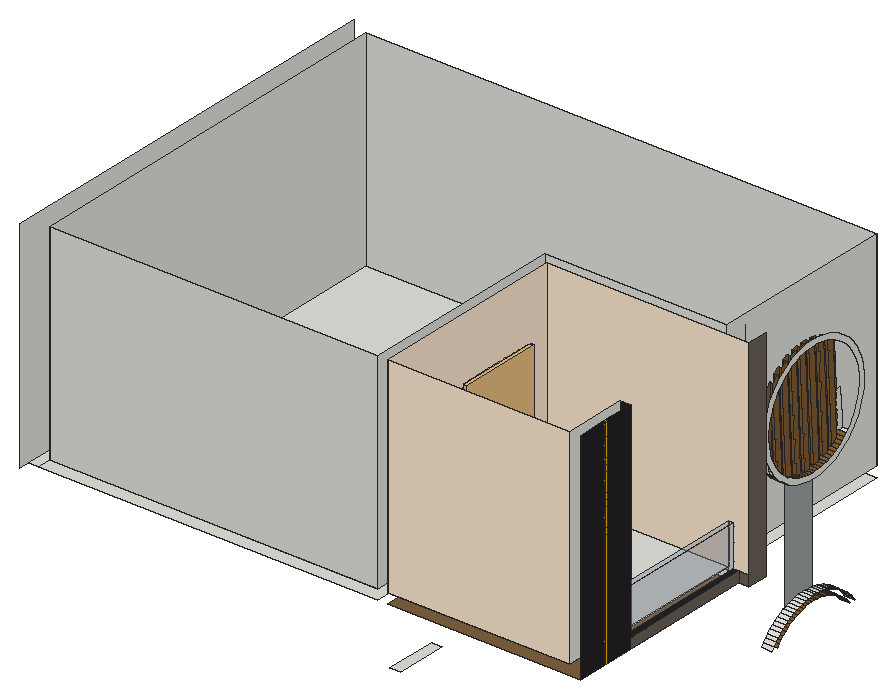
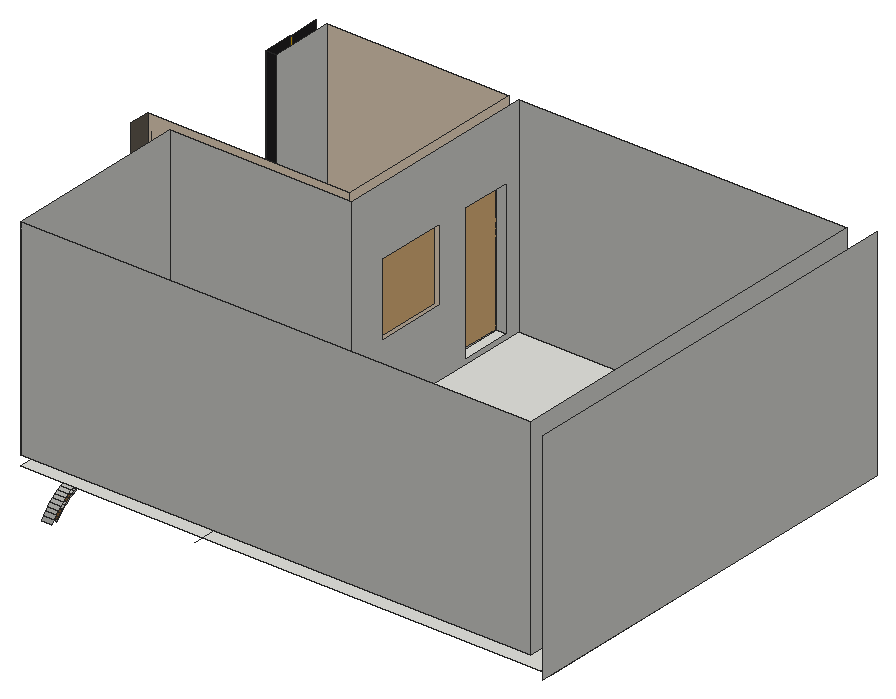
# SketchUp Ruby script. Lengths in inches.
U = 1.inch
M = Sketchup.active_model
def pt(a) = Geom::Point3d.new(a.map { |v| v * U })
def face(e, loops, mat)
  f = e.add_face(loops[0].map { |a| pt(a) })
  loops[1..].each { |l| e.add_face(l.map { |a| pt(a) }).erase! }
  f.material = f.back_material = mat if mat
  f
end
# faces: each face lists its corners as indices into pts; further lists are holes
def faces(e, pts, list, mat = nil) = list.each { |f| face(e, (f[0].is_a?(Array) ? f : [f]).map { |l| l.map { |i| pts[i] } }, mat) }
# xy, xz, yz: faces in a plane at the given z, y or x. An outline is a flat list of corners, or four numbers for a rectangle; further outlines are holes
def ring(l) = l.size == 4 ? [[l[0], l[1]], [l[2], l[1]], [l[2], l[3]], [l[0], l[3]]] : l.each_slice(2).to_a
def flat(e, list, mat, &to3) = list.each { |f| face(e, (f[0].is_a?(Array) ? f : [f]).map { |l| ring(l).map { |u, v| to3.(u, v) } }, mat) }
def xy(e, z, list, mat = nil) = flat(e, list, mat) { |x, y| [x, y, z] }
def xz(e, y, list, mat = nil) = flat(e, list, mat) { |x, z| [x, y, z] }
def yz(e, x, list, mat = nil) = flat(e, list, mat) { |y, z| [x, y, z] }
def lines(e, pts, list) = list.each { |a, b| e.add_line(pt(pts[a]), pt(pts[b])) }
# prism: a flat outline (further loops are holes) pulled along v
def prism(e, loops, v, mat = nil)
  f = face(e, loops, mat); d = Geom::Vector3d.new(v.map { |x| x * U })
  f.pushpull(f.normal.samedirection?(d) ? d.length : -d.length)
end
def box(e, o, s, mat = nil) = prism(e, [[o, [o[0] + s[0], o[1], o[2]], [o[0] + s[0], o[1] + s[1], o[2]], [o[0], o[1] + s[1], o[2]]]], [0, 0, s[2]], mat)
def at(x, y, z, deg = 0) = Geom::Transformation.translation(pt([x, y, z])) * Geom::Transformation.rotation(ORIGIN, Z_AXIS, deg.degrees)
def axes(o, x, y, z) = Geom::Transformation.new([*x, 0, *y, 0, *z, 0, *pt(o).to_a, 1])
def part(name) = M.definitions.add(name)
# library, detail: a bought-in or finely detailed component or shape, given as its bounding box
def library(name, o, s) = part(name).tap { |d| box(d.entities, o, s) }
def detail(e, o, s) = box(e.add_group.entities, o, s)
def put(e, d, t, mat = nil) = e.add_instance(d, t).tap { |i| i.material = mat if mat }
def group(e, t, mat = nil) = e.add_group.tap { |g| g.transformation = t; g.material = mat if mat }.entities
root = M.entities
M.materials.add("C03_Honey_Glow").color = [255, 234, 209]
M.materials.add("C08_Toffee_Ember").color = [130, 92, 50]
M.materials.add("D05_Goldenrod_Hue").color = [255, 191, 0]
M.materials.add("Denim_03_1K").color = [156, 160, 160]
M.materials.add("Glass_Basic_01").color = [161, 173, 186]
M.materials["Glass_Basic_01"].alpha = 0.25
M.materials.add("Marble_07_1K").color = [36, 34, 36]
M.materials.add("Plaster_04_1K").color = [106, 98, 87]
M.materials.add("Plywood_01_1K").color = [125, 96, 64]
c1 = library("porta+4",[0.2,-5.42,1.33],[46.55,4.72,83.21])
c2 = library("mesh-165",[-1596.32,-2661.67,-39.91],[1702.88,1739.15,82.5])
c3 = part("Group15")
put(c3.entities,c2,at(294.66,859.51,3.5))
xy(root,213,[[206.5,30,212.5,60],[206.5,78,212.5,120]])
xy(root,252,[[5.5,21,11.5,135],[11.5,21,206.5,249],[317.82,101.57,320.5,104.14],[317.82,106.71,320.5,109.29],[317.82,111.86,320.5,114.43],
  [317.5,117,320.5,119.57],[317.5,122.14,320.5,124.71],[317.5,127.29,320.5,129.86],[317.5,132.43,320.5,135],[5.5,135,11.5,249],
  [206.5,135,317.5,141],[206.5,141,311.5,249]])
xy(root,252,[[[212.5,21,212.5,135,317.5,135,317.5,132.43,320.5,132.43,320.5,135,323.5,135,323.5,21],[317.82,101.57,320.5,101.57,320.5,104.14,317.82,104.14,317.82,106.71,320.5,106.71,320.5,109.29,317.82,109.29,317.82,111.86,320.5,111.86,320.5,114.43,317.82,114.43],[317.5,127.29,320.5,129.86],[317.5,122.14,320.5,124.71],[317.5,117,320.5,119.57]]],"Plywood_01_1K")
xy(root,258,[[17.5,21,206.67,21,206.67,141,311.5,141,311.5,249,17.5,249],[212.67,21,317.5,135]])
xy(root,258,[[320.5,57,323.5,135]],"Marble_07_1K")
xy(root,261,[[206.67,30,212.67,60]])
xy(root,282,[[317.5,57,320.5,135]],"Glass_Basic_01")
xz(root,21,[[17.5,258,206.67,378]])
xz(root,21,[[212.67,258,317.5,378]],"C03_Honey_Glow")
xz(root,30,[[206.67,261,212.67,339]])
xz(root,57,[[320.5,258,323.5,282],[317.5,282,323.5,378]],"Marble_07_1K")
xz(root,60,[[206.67,261,212.67,339]])
xz(root,135,[[317.5,252,320.5,282],[320.5,252,323.5,258]])
xz(root,135,[[212.67,258,317.5,258,317.5,282,320.5,282,320.5,258,329.5,258,329.5,378,212.67,378]],"C03_Honey_Glow")
xz(root,135,[[323.5,252,329.5,258]],"Plaster_04_1K")
xz(root,141,[[206.67,258,311.5,378]])
xz(root,249,[[17.5,258,311.5,378]])
yz(root,5.5,[[15,252,255,378]])
yz(root,17.5,[[21,258,249,378]])
yz(root,206.67,[[[21,258,141,378],[30,261,60,339],[78,297,120,339]]])
yz(root,212.67,[[[27,258,63,342],[30,261,60,339]],[[75,294,123,342],[78,297,120,339]]])
yz(root,212.67,[[[21,258,27,258,27,342,63,342,63,258,135,258,135,378,21,378],[75,294,123,342]]],"C03_Honey_Glow")
yz(root,311.5,[[141,258,249,378]])
yz(root,317.5,[[214.37,207.08,214.35,207.56,213.31,208.76,211.86,210.24,210.86,211.15,210.88,210.69,212.14,209.53,213.57,208.03],[164.74,208.35,165.47,209.14,166.97,210.57,167.89,211.34,167.87,211.77,166.68,210.75,165.2,209.3,164.72,208.77],[210.88,210.69,210.86,211.15,210.32,211.63,208.7,212.92,207.41,213.8125,207.4375,213.36,209.01,212.24,210.61,210.9375],[167.89,211.34,168.55,211.9,170.22,213.14,171.07,213.6875,171.05,214.12,169.91,213.36,168.25,212.11,167.87,211.77],[207.4375,213.36,207.41,213.8125,207,214.11,205.22,215.18,204.01,215.82,204.03,215.37,205.56,214.55,207.32,213.45],
  [171.07,213.6875,171.96,214.26,173.77,215.28,174.28,215.52,174.26,215.95,173.43,215.54,171.63,214.5,171.05,214.12],[204.03,215.37,204.01,215.82,203.39,216.14,201.49,216.99,200.625,217.3125,200.65,216.86,201.85,216.4,203.73,215.53],[174.28,215.52,175.64,216.17,177.51,216.93,177.49,217.36,177.2,217.26,175.29,216.46,174.26,215.95],[200.65,216.86,200.625,217.3125,199.55,217.71,197.57,218.3125,197.27,218.38,197.29,217.93,197.9375,217.77,199.92,217.14],[177.51,216.93,177.56,216.95,179.53,217.61,180.77,217.94,180.74,218.38,179.16,217.94,177.49,217.36],
  [197.29,217.93,197.27,218.38,195.55,218.79,194.92,218.9,194.92,218.45,195.93,218.26],[180.77,217.94,181.53,218.14,183.5625,218.55,184.04,218.61,184.01,219.05,183.18,218.93,181.15,218.5,180.74,218.38],[194.92,218.45,194.92,218.9,193.93,219.0625,193.95,218.625],[184.04,218.61,185.62,218.83,187.32,218.95,187.3,219.4,185.23,219.23,184.01,219.05],[193.95,218.625,193.93,219.0625,193.51,219.14,191.44,219.35,190.6,219.39,190.63,218.94,191.83,218.88,193.89,218.64],
  [190.63,218.94,190.6,219.39,189.37,219.44,187.3,219.4,187.32,218.95,187.69,218.97,189.76,218.99],[21,258,57,378],[207.125,286.92,207.95,287.39,209.83,288.64,210.32,289.01,210.13,292.67,208.96,315.33,205.66,315.33,206.95,290.33],[170.77,286.97,170.59,290.63,169.3125,315.33,166.01,315.33,167.14,293.29,167.35,289.24,167.51,289.12,169.37,287.82],[213.49,291.625,214.96,293.0625,216.48,294.74,216.625,294.93,216.38,299.61,215.57,315.33,212.27,315.33,213.28,295.68],
  [163.9,292.21,163.65,296.89,162.7,315.33,159.4,315.33,160.08,302.125,160.39,296.18,161,295.37,162.48,293.65]])
yz(root,317.5,[[190.7,285.04,192.77,285.22,193.99,285.39,192.44,315.33,190.6,350.95,189.37,351,187.3,350.96,189.14,315.33],[187.4,285.05,185.83,315.33,184.01,350.61,183.18,350.48,181.15,350.05,180.74,349.9375,182.53,315.33,184.07,285.38,184.49,285.31,186.56,285.09],[180.73,286.06,179.22,315.33,177.49,348.92,177.2,348.82,175.29,348.02,174.26,347.51,175.92,315.33,177.375,287.13,178.45,286.73,180.43,286.13],[197.26,286.0625,198.84,286.5,200.51,287.08,199.05,315.33,197.27,349.94,195.55,350.34,194.92,350.45,194.92,331.43,195.75,315.33],[203.74,288.49,204.57,288.9,206.37,289.9375,206.95,290.33,205.66,315.33,204.01,347.375,203.39,347.7,201.49,348.54,200.625,348.87,202.36,315.33],
  [173.99,288.625,172.62,315.33,171.05,345.67,169.91,344.91,168.25,343.66,167.87,343.33,169.3125,315.33,170.59,290.63,171,290.34,172.78,289.26],[210.13,292.67,211.32,293.69,212.8,295.14,213.28,295.68,212.27,315.33,210.86,342.71,210.32,343.1875,208.7,344.48,207.41,345.37,208.96,315.33],[167.14,293.29,166.01,315.33,164.72,340.32,163.8125,339.32,162.52,337.7,161.62,336.39,162.7,315.33,163.65,296.89,164.69,295.68,166.14,294.2]],"C08_Toffee_Ember")
yz(root,317.5,[[175.37,219.3,176.52,219.77,178.67,220.48,180.85,221.07,183.07,221.51,185.31,221.81,187.57,221.97,189.83,221.99,192.09,221.87,194.33,221.6,194.92,221.5,194.92,282.5,193.11,282.24,190.86,282.05,188.59,282,186.33,282.1,184.09,282.34,181.86,282.72,179.65,283.23,177.49,283.89,175.37,284.68]],"Denim_03_1K")
yz(root,317.5,[[57,258,135,282]],"Glass_Basic_01")
yz(root,319.5,[[188.63,285,190.7,285.04,187.3,350.96,185.23,350.78,184.01,350.61,187.4,285.05],[184.07,285.38,180.74,349.9375,179.16,349.5,177.49,348.92,180.73,286.06,182.45,285.66],[193.99,285.39,194.82,285.52,196.85,285.95,197.26,286.0625,193.93,350.62,193.51,350.69,191.44,350.91,190.6,350.95],[200.51,287.08,200.8,287.18,202.71,287.98,203.74,288.49,200.625,348.87,199.55,349.27,197.57,349.87,197.27,349.94],[177.375,287.13,174.26,347.51,173.43,347.1,171.63,346.0625,171.05,345.67,173.99,288.625,174.61,288.3,176.51,287.46],
  [206.95,290.33,208.09,291.09,209.75,292.34,210.13,292.67,207.41,345.37,207,345.66,205.22,346.74,204.01,347.375],[170.59,290.63,167.87,343.33,166.68,342.31,165.2,340.86,164.72,340.32,167.14,293.29,167.68,292.8125,169.3,291.52]],"C08_Toffee_Ember")
yz(root,320.5,[[57,258,135,282]],"Glass_Basic_01")
yz(root,323.5,[[[188.59,282,190.86,282.05,193.11,282.24,195.35,282.5625,197.56,283.03,199.74,283.64,201.875,284.38,203.96,285.26,205.99,286.26,207.95,287.39,209.83,288.64,211.63,290,213.35,291.48,214.96,293.0625,216.48,294.74,217.88,296.51,219.18,298.37,220.35,300.3,221.4,302.31,222.32,304.37,223.11,306.49,223.77,308.65,224.28,310.86,224.66,313.09,224.9,315.33,225,317.59,224.95,319.86,224.76,322.11,224.4375,324.35,223.97,326.56,223.36,328.74,222.62,330.875,221.74,332.96,220.74,334.99,219.61,336.95,218.36,338.83,217,340.63,215.52,342.35,213.9375,343.96,212.26,345.48,210.49,346.88,208.63,348.18,206.7,349.35,204.69,350.4,202.63,351.32,200.51,352.11,198.35,352.77,196.14,353.28,193.91,353.66,191.67,353.9,189.41,354,187.14,353.95,184.89,353.76,182.65,353.4375,180.44,352.97,178.26,352.36,176.125,351.62,174.04,350.74,172.01,349.74,170.05,348.61,168.17,347.36,166.37,346,164.65,344.52,163.04,342.9375,161.52,341.26,160.12,339.49,158.82,337.63,157.65,335.7,156.6,333.69,155.68,331.63,154.89,329.51,154.23,327.35,153.72,325.14,153.34,322.91,153.1,320.67,153,318.41,153.05,316.14,153.24,313.89,153.5625,311.65,154.03,309.44,154.64,307.26,155.38,305.125,156.26,303.04,157.26,301.01,158.39,299.05,159.64,297.17,161,295.37,162.48,293.65,164.0625,292.04,165.74,290.52,167.51,289.12,169.37,287.82,171.3,286.65,173.31,285.6,175.37,284.68,177.49,283.89,179.65,283.23,181.86,282.72,184.09,282.34,186.33,282.1],[188.63,285,186.56,285.09,184.49,285.31,182.45,285.66,180.43,286.13,178.45,286.73,176.51,287.46,174.61,288.3,172.78,289.26,171,290.34,169.3,291.52,167.68,292.8125,166.14,294.2,164.69,295.68,163.34,297.25,162.09,298.91,160.9375,300.63,159.9,302.43,158.98,304.29,158.18,306.2,157.5,308.16,156.95,310.15,156.52,312.18,156.22,314.23,156.04,316.3,156,318.37,156.09,320.44,156.31,322.51,156.66,324.55,157.13,326.57,157.73,328.55,158.46,330.49,159.3,332.39,160.26,334.22,161.34,336,162.52,337.7,163.8125,339.32,165.2,340.86,166.68,342.31,168.25,343.66,169.91,344.91,171.63,346.0625,173.43,347.1,175.29,348.02,177.2,348.82,179.16,349.5,181.15,350.05,183.18,350.48,185.23,350.78,187.3,350.96,189.37,351,191.44,350.91,193.51,350.69,195.55,350.34,197.57,349.87,199.55,349.27,201.49,348.54,203.39,347.7,205.22,346.74,207,345.66,208.7,344.48,210.32,343.1875,211.86,341.8,213.31,340.32,214.66,338.75,215.91,337.09,217.0625,335.37,218.1,333.57,219.02,331.71,219.82,329.8,220.5,327.84,221.05,325.85,221.48,323.82,221.78,321.77,221.96,319.7,222,317.63,221.91,315.56,221.69,313.49,221.34,311.45,220.87,309.43,220.27,307.45,219.54,305.51,218.7,303.61,217.74,301.78,216.66,300,215.48,298.3,214.1875,296.68,212.8,295.14,211.32,293.69,209.75,292.34,208.09,291.09,206.37,289.9375,204.57,288.9,202.71,287.98,200.8,287.18,198.84,286.5,196.85,285.95,194.82,285.52,192.77,285.22,190.7,285.04]]])
yz(root,323.5,[[38,252,39,378],[39,252,40,378]],"D05_Goldenrod_Hue")
yz(root,323.5,[[21,252,38,378],[40,252,57,378]],"Marble_07_1K")
yz(root,323.5,[[57,252,135,258]],"Plaster_04_1K")
yz(root,329.5,[[135,252,147,378]],"Plaster_04_1K")
p = [[317.5,160.37,207.82],[317.5,159.06,205.98],[323.5,159.06,205.98],[323.5,160.37,207.82],[317.5,162.76,206.01],[317.5,164.0625,207.61],
  [319.5,164.0625,207.61],[319.5,162.76,206.01],[323.5,162.76,206.01],[323.5,164.0625,207.61],[317.5,213.57,208.03],[317.5,214.37,207.08],
  [319.5,214.37,207.08],[319.5,214.9,206.45],[323.5,214.9,206.45],[323.5,213.57,208.03],[317.5,214.9,206.45],[317.5,218.6,206.49],
  [317.5,217.26,208.3],[323.5,217.26,208.3],[323.5,218.6,206.49],[319.5,164.74,208.35],[317.5,164.74,208.35],[317.5,165.47,209.14],
  [323.5,165.47,209.14],[317.5,161.8,209.58],[323.5,161.8,209.58],[317.5,212.14,209.53],[323.5,212.14,209.53],[317.5,215.8,210.03],
  [323.5,215.8,210.03],[317.5,166.97,210.57],[323.5,166.97,210.57],[323.5,210.61,210.9375],[319.5,210.61,210.9375],[319.5,210.88,210.69],
  [317.5,210.88,210.69],[317.5,163.33,211.24],[323.5,163.33,211.24],[317.5,214.24,211.67],[323.5,214.24,211.67],[317.5,167.89,211.34],
  [319.5,167.89,211.34],[319.5,168.55,211.9],[323.5,168.55,211.9],[317.5,210.61,210.9375],[317.5,209.01,212.24],[319.5,209.01,212.24],
  [323.5,209.01,212.24],[317.5,164.97,212.8],[323.5,164.97,212.8],[317.5,168.55,211.9],[317.5,212.58,213.2],[323.5,212.58,213.2],
  [317.5,170.22,213.14],[319.5,170.22,213.14],[323.5,170.22,213.14],[317.5,207.32,213.45],[317.5,207.4375,213.36],[319.5,207.4375,213.36],
  [323.5,207.32,213.45],[317.5,166.7,214.26],[323.5,166.7,214.26],[319.5,171.07,213.6875],[317.5,171.07,213.6875],[317.5,171.96,214.26],
  [323.5,171.96,214.26],[317.5,210.82,214.63],[323.5,210.82,214.63],[317.5,205.56,214.55],[323.5,205.56,214.55],[317.5,168.51,215.6],
  [323.5,168.51,215.6],[317.5,173.77,215.28],[323.5,173.77,215.28],[323.5,203.73,215.53],[319.5,203.73,215.53],[319.5,204.03,215.37],
  [317.5,204.03,215.37],[317.5,208.98,215.94],[323.5,208.98,215.94],[317.5,174.28,215.52],[319.5,174.28,215.52],[319.5,175.64,216.17],
  [323.5,175.64,216.17],[317.5,203.73,215.53],[317.5,175.64,216.17],[317.5,201.85,216.4],[319.5,201.85,216.4],[323.5,201.85,216.4],
  [317.5,170.41,216.83],[323.5,170.41,216.83],[317.5,207.0625,217.14],[323.5,207.0625,217.14],[319.5,177.51,216.93],[317.5,177.51,216.93],
  [317.5,177.56,216.95],[323.5,177.56,216.95],[317.5,199.92,217.14],[317.5,200.65,216.86],[319.5,200.65,216.86],[323.5,199.92,217.14],
  [317.5,172.39,217.9375],[323.5,172.39,217.9375],[317.5,179.53,217.61],[323.5,179.53,217.61],[317.5,197.9375,217.77],[323.5,197.9375,217.77],
  [317.5,205.07,218.21],[323.5,205.07,218.21],[317.5,180.77,217.94],[319.5,180.77,217.94],[319.5,181.53,218.14],[323.5,181.53,218.14],
  [323.5,195.93,218.26],[319.5,195.93,218.26],[319.5,197.29,217.93],[317.5,197.29,217.93],[317.5,174.42,218.92],[323.5,174.42,218.92],
  [317.5,181.53,218.14],[317.5,195.93,218.26],[317.5,183.5625,218.55],[319.5,183.5625,218.55],[323.5,183.5625,218.55],[317.5,203.02,219.16],
  [323.5,203.02,219.16],[317.5,193.89,218.64],[317.5,193.95,218.625],[319.5,193.95,218.625],[323.5,193.89,218.64],[317.5,194.92,218.45],
  [319.5,184.04,218.61],[317.5,184.04,218.61],[317.5,185.62,218.83],[323.5,185.62,218.83],[317.5,191.83,218.88],[323.5,191.83,218.88],
  [317.5,187.32,218.95],[319.5,187.32,218.95],[319.5,187.69,218.97],[323.5,187.69,218.97],[317.5,175.37,219.3],[323.5,176.52,219.77],
  [317.5,176.52,219.77],[317.5,187.69,218.97],[323.5,189.76,218.99],[319.5,189.76,218.99],[319.5,190.63,218.94],[317.5,190.63,218.94],
  [317.5,189.76,218.99],[317.5,200.91,219.97],[323.5,200.91,219.97],[317.5,178.67,220.48],[323.5,178.67,220.48],[317.5,198.75,220.65],
  [323.5,198.75,220.65],[317.5,180.85,221.07],[323.5,180.85,221.07],[317.5,196.56,221.2],[323.5,196.56,221.2],[317.5,183.07,221.51],
  [323.5,183.07,221.51],[317.5,194.92,221.5],[317.5,194.33,221.6],[323.5,194.33,221.6],[317.5,185.31,221.81],[323.5,185.31,221.81],
  [317.5,192.09,221.87],[323.5,192.09,221.87],[317.5,187.57,221.97],[323.5,187.57,221.97],[317.5,189.83,221.99],[323.5,189.83,221.99],
  [317.5,186.33,282.1],[317.5,188.59,282],[323.5,188.59,282],[323.5,186.33,282.1],[317.5,190.86,282.05],[323.5,190.86,282.05],
  [317.5,193.11,282.24],[323.5,193.11,282.24],[317.5,184.09,282.34],[323.5,184.09,282.34],[317.5,194.92,282.5],[317.5,195.35,282.5625],
  [323.5,195.35,282.5625],[317.5,181.86,282.72],[323.5,181.86,282.72],[317.5,197.56,283.03],[323.5,197.56,283.03],[317.5,179.65,283.23],
  [323.5,179.65,283.23],[317.5,199.74,283.64],[323.5,199.74,283.64],[317.5,177.49,283.89],[323.5,177.49,283.89],[317.5,201.875,284.38],
  [323.5,201.875,284.38],[317.5,175.37,284.68],[323.5,175.37,284.68],[317.5,203.96,285.26],[323.5,203.96,285.26],[317.5,174.17,285.22],
  [323.5,173.31,285.6],[317.5,173.31,285.6],[323.5,188.63,285],[319.5,188.63,285],[319.5,187.4,285.05],[317.5,187.4,285.05],
  [317.5,186.56,285.09],[323.5,186.56,285.09],[317.5,189.14,315.33],[317.5,187.3,350.96],[319.5,187.3,350.96],[319.5,190.7,285.04],
  [317.5,190.7,285.04],[323.5,190.7,285.04],[317.5,192.77,285.22],[323.5,192.77,285.22],[317.5,184.01,350.61],[317.5,185.83,315.33],
  [319.5,184.01,350.61],[317.5,184.49,285.31],[323.5,184.49,285.31],[323.5,194.82,285.52],[319.5,194.82,285.52],[319.5,193.99,285.39],
  [317.5,193.99,285.39],[317.5,184.07,285.38],[319.5,184.07,285.38],[319.5,182.45,285.66],[323.5,182.45,285.66],[317.5,205.99,286.26],
  [323.5,205.99,286.26],[317.5,182.53,315.33],[317.5,180.74,349.9375],[319.5,180.74,349.9375],[317.5,190.6,350.95],[317.5,192.44,315.33],
  [319.5,190.6,350.95],[323.5,196.85,285.95],[319.5,196.85,285.95],[317.5,171.3,286.65],[323.5,171.3,286.65],[319.5,180.73,286.06],
  [317.5,180.73,286.06],[317.5,180.43,286.13],[323.5,180.43,286.13],[317.5,198.84,286.5],[317.5,197.26,286.0625],[319.5,197.26,286.0625],
  [323.5,198.84,286.5],[317.5,177.49,348.92],[317.5,179.22,315.33],[319.5,177.49,348.92],[317.5,178.45,286.73],[323.5,178.45,286.73],
  [317.5,194.92,331.43],[317.5,193.93,350.62],[319.5,193.93,350.62],[317.5,195.75,315.33],[317.5,207.125,286.92],[317.5,207.95,287.39],
  [323.5,207.95,287.39],[323.5,200.8,287.18],[319.5,200.8,287.18],[319.5,200.51,287.08],[317.5,200.51,287.08],[317.5,170.77,286.97],
  [323.5,169.37,287.82],[317.5,169.37,287.82],[317.5,177.375,287.13],[319.5,177.375,287.13],[319.5,176.51,287.46],[323.5,176.51,287.46],
  [317.5,175.92,315.33],[317.5,174.26,347.51],[319.5,174.26,347.51],[317.5,197.27,349.94],[317.5,199.05,315.33],[319.5,197.27,349.94],
  [323.5,202.71,287.98],[319.5,202.71,287.98],[317.5,209.83,288.64],[323.5,209.83,288.64],[319.5,174.61,288.3],[323.5,174.61,288.3],
  [317.5,167.51,289.12],[323.5,167.51,289.12],[317.5,204.57,288.9],[317.5,203.74,288.49],[319.5,203.74,288.49],[323.5,204.57,288.9],
  [319.5,173.99,288.625],[317.5,173.99,288.625],[317.5,172.78,289.26],[323.5,172.78,289.26],[317.5,202.36,315.33],[317.5,200.625,348.87],
  [319.5,200.625,348.87],[317.5,171.05,345.67],[317.5,172.62,315.33],[319.5,171.05,345.67],[317.5,210.32,289.01],[317.5,211.63,290],
  [323.5,211.63,290],[317.5,206.37,289.9375],[323.5,206.37,289.9375],[317.5,167.35,289.24],[323.5,165.74,290.52],[317.5,165.74,290.52],
  [317.5,171,290.34],[323.5,171,290.34],[323.5,208.09,291.09],[319.5,208.09,291.09],[319.5,206.95,290.33],[317.5,206.95,290.33],
  [317.5,213.35,291.48],[323.5,213.35,291.48],[317.5,170.59,290.63],[319.5,170.59,290.63],[319.5,169.3,291.52],[323.5,169.3,291.52],
  [317.5,204.01,347.375],[317.5,205.66,315.33],[319.5,204.01,347.375],[317.5,164.0625,292.04],[323.5,164.0625,292.04],[317.5,169.3125,315.33],
  [317.5,167.87,343.33],[319.5,167.87,343.33],[323.5,209.75,292.34],[319.5,209.75,292.34],[319.5,167.68,292.8125],[323.5,167.68,292.8125],
  [317.5,213.49,291.625],[317.5,214.96,293.0625],[323.5,214.96,293.0625],[317.5,163.9,292.21],[323.5,162.48,293.65],[317.5,162.48,293.65],
  [317.5,211.32,293.69],[317.5,210.13,292.67],[319.5,210.13,292.67],[323.5,211.32,293.69],[317.5,208.96,315.33],[317.5,207.41,345.37],
  [319.5,207.41,345.37],[319.5,167.14,293.29],[317.5,167.14,293.29],[317.5,166.14,294.2],[323.5,166.14,294.2],[317.5,216.48,294.74],
  [323.5,216.48,294.74],[317.5,164.72,340.32],[317.5,166.01,315.33],[319.5,164.72,340.32],[317.5,161,295.37],[323.5,161,295.37],
  [317.5,212.8,295.14],[323.5,212.8,295.14],[317.5,164.69,295.68],[323.5,164.69,295.68],[206.5,249,252],[206.5,255,252],
  [317.5,132.43,252],[317.5,129.86,252],[317.5,127.29,252],[317.5,124.71,252],[317.5,122.14,252],[317.5,119.57,252],
  [317.5,117,252],[317.5,114.43,252],[317.5,194,285.21],[317.5,197.29,285.38],[317.5,200.59,285.55],[317.5,203.88,285.72],
  [317.5,187.4,284.875],[317.5,184.11,284.7],[317.5,180.8125,284.53],[317.5,177.52,284.36],[317.5,194.92,218.9],[317.5,194.92,315.33],
  [317.5,141,252],[317.5,146.83,252],[317.5,146.83,378],[317.5,147,252]]
faces(root,p,[[0,1,2,3],[4,5,6,7],[11,16,13,12],[17,18,19,20],[5,22,21,6],[25,0,3,26],[18,29,30,19],[37,25,26,38],
  [29,39,40,30],[45,36,35,34],[46,45,34,47],[49,37,38,50],[41,51,43,42],[39,52,53,40],[51,54,55,43],[58,46,47,59],
  [61,49,50,62],[54,64,63,55],[52,67,68,53],[71,61,62,72],[67,79,80,68],[85,78,77,76],[81,86,83,82],[87,85,76,88],
  [90,71,72,91],[79,92,93,80],[86,95,94,83],[99,87,88,100],[102,90,91,103],[92,108,109,93],[118,102,103,119],[110,120,112,111],
  [121,117,116,115],[120,122,123,112],[108,125,126,109],[128,131,121,115,129],[122,133,132,123],[142,118,119,143,144],[138,145,140,139],[150,149,148,147],
  [145,150,147,140],[125,151,152,126],[153,144,143,154],[151,155,156,152],[157,153,154,158],[155,159,160,156],[161,157,158,162],[163,164,165,160,159],
  [166,161,162,167],[164,168,169,165],[170,166,167,171],[168,172,173,169],[172,170,171,173],[174,175,176,177],[175,178,179,176],[178,180,181,179],
  [182,174,177,183],[184,185,186,181,180],[187,182,183,188],[185,189,190,186],[191,187,188,192],[189,193,194,190],[195,191,192,196],[193,197,198,194],
  [199,195,196,200],[197,201,202,198],[203,199,200,204,205],[201,233,234,202],[243,205,204,244],[262,263,264,234,233],[269,243,244,270,271],[263,284,285,264],
  [288,271,270,289],[304,305,306,285,284],[309,288,289,310,311],[305,318,319,306],[327,311,310,328],[336,337,338,319,318],[339,327,328,340,341],[337,353,354,338],
  [358,341,340,359]])
faces(root,p,[[8,7,6,9],[10,11,12,13,14,15],[9,6,21,22,23,24],[27,10,15,28],[23,31,32,24],[33,34,35,36,27,28],[31,41,42,43,44,32],[48,47,34,33],
  [44,43,55,56],[57,58,59,47,48,60],[56,55,63,64,65,66],[69,57,60,70],[65,73,74,66],[75,76,77,78,69,70],[73,81,82,83,84,74],[89,88,76,75],
  [84,83,94,95,96,97],[98,99,100,88,89,101],[96,104,105,97],[106,98,101,107],[104,110,111,112,113,105],[114,115,116,117,106,107],[113,112,123,124],[127,128,129,115,114,130],
  [124,123,132,133,134,135],[136,127,130,137],[134,138,139,140,141,135],[146,147,148,149,136,137],[141,140,147,146],[206,207,208,209,210,211],[212,213,214,215,216],[217,215,207,206],
  [218,216,215,217,219],[220,221,209,208,222],[210,223,224,211],[225,226,227,228,218,219],[223,229,230,231,232,224],[235,236,237,230,229],[238,239,228,227,240],[241,242,226,225],
  [232,231,245,246,247,248],[249,250,251,242,241,252],[253,254,246,245,255],[247,256,257,248],[258,259,260,251,250,261],[265,266,267,268,249,252],[256,272,273,274,275,257],[276,277,278,273,272],
  [279,280,268,267,281],[282,283,266,265],[275,274,286,287],[290,291,292,283,282,293],[287,286,294,295,296,297],[298,299,300,292,291],[301,302,295,294,303],[307,290,293,308],
  [296,312,313,297],[314,315,316,317,307,308],[312,320,321,322,323,313],[324,325,317,316,326],[329,330,331,321,320],[332,333,315,314],[323,322,334,335],[342,343,344,333,332,345],
  [346,347,348,344,343],[335,334,349,350,351,352],[355,356,350,349,357],[360,342,345,361],[351,362,363,352]],"C08_Toffee_Ember")
lines(root,p,[[364,365],[366,367],[368,369],[370,371],[372,373],[228,374],[250,375],[268,376],[291,377],[209,378],[229,379],[246,380],
  [272,381],[295,203],[382,163],[184,383],[384,385],[385,386],[385,387]])
put(root,c1,axes([211.97,26.84,256.67],[0,0.77339,0],[-1,0,0],[0,0,1]))
put(root,c3,axes([213.9375,86.28,343.74],[0,-0.02811,0],[0,0,0.02756],[-0.02756,0,0]))
